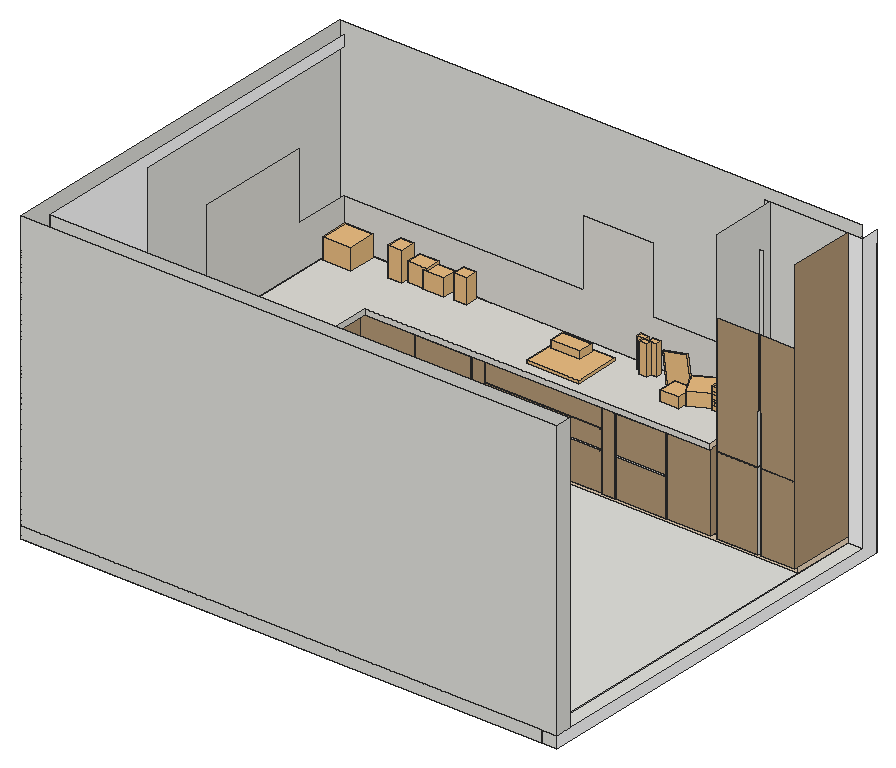
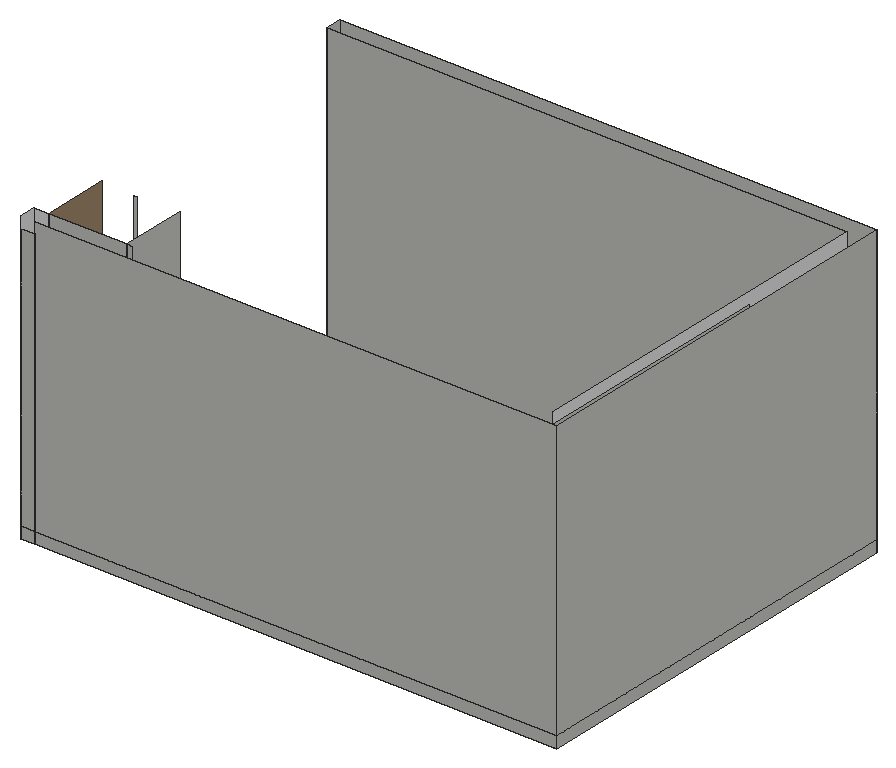
# SketchUp Ruby script. Lengths in inches.
U = 1.inch
M = Sketchup.active_model
def pt(a) = Geom::Point3d.new(a.map { |v| v * U })
def face(e, loops, mat)
  f = e.add_face(loops[0].map { |a| pt(a) })
  loops[1..].each { |l| e.add_face(l.map { |a| pt(a) }).erase! }
  f.material = f.back_material = mat if mat
  f
end
# faces: each face lists its corners as indices into pts; further lists are holes
def faces(e, pts, list, mat = nil) = list.each { |f| face(e, (f[0].is_a?(Array) ? f : [f]).map { |l| l.map { |i| pts[i] } }, mat) }
# xy, xz, yz: faces in a plane at the given z, y or x. An outline is a flat list of corners, or four numbers for a rectangle; further outlines are holes
def ring(l) = l.size == 4 ? [[l[0], l[1]], [l[2], l[1]], [l[2], l[3]], [l[0], l[3]]] : l.each_slice(2).to_a
def flat(e, list, mat, &to3) = list.each { |f| face(e, (f[0].is_a?(Array) ? f : [f]).map { |l| ring(l).map { |u, v| to3.(u, v) } }, mat) }
def xy(e, z, list, mat = nil) = flat(e, list, mat) { |x, y| [x, y, z] }
def xz(e, y, list, mat = nil) = flat(e, list, mat) { |x, z| [x, y, z] }
def yz(e, x, list, mat = nil) = flat(e, list, mat) { |y, z| [x, y, z] }
def lines(e, pts, list) = list.each { |a, b| e.add_line(pt(pts[a]), pt(pts[b])) }
# prism: a flat outline (further loops are holes) pulled along v
def prism(e, loops, v, mat = nil)
  f = face(e, loops, mat); d = Geom::Vector3d.new(v.map { |x| x * U })
  f.pushpull(f.normal.samedirection?(d) ? d.length : -d.length)
end
def box(e, o, s, mat = nil) = prism(e, [[o, [o[0] + s[0], o[1], o[2]], [o[0] + s[0], o[1] + s[1], o[2]], [o[0], o[1] + s[1], o[2]]]], [0, 0, s[2]], mat)
def at(x, y, z, deg = 0) = Geom::Transformation.translation(pt([x, y, z])) * Geom::Transformation.rotation(ORIGIN, Z_AXIS, deg.degrees)
def axes(o, x, y, z) = Geom::Transformation.new([*x, 0, *y, 0, *z, 0, *pt(o).to_a, 1])
def part(name) = M.definitions.add(name)
# library, detail: a bought-in or finely detailed component or shape, given as its bounding box
def library(name, o, s) = part(name).tap { |d| box(d.entities, o, s) }
def detail(e, o, s) = box(e.add_group.entities, o, s)
def put(e, d, t, mat = nil) = e.add_instance(d, t).tap { |i| i.material = mat if mat }
def group(e, t, mat = nil) = e.add_group.tap { |g| g.transformation = t; g.material = mat if mat }.entities
root = M.entities
M.materials.add("Generic").color = [180, 152, 118]
M.materials.add("Generic\#2").color = [244, 221, 193]
M.materials.add("Sink Modena 7170-03").color = [86, 64, 57]
M.materials.add("[Color M00]").color = [255, 255, 255]
M.materials.add("[Marble Carrara Gold Floor Tile]").color = [224, 222, 216]
M.materials.add("besi putih_Glossy3").color = [240, 240, 240]
M.materials.add("go trang").color = [128, 128, 128]
c1 = library("Group\#102",[0,0,-8.66],[20.47,15.75,8.66])
c2 = library("itchenFaucet_Handspray\#1",[0.83,4.01,0],[10.6,4,15.3])
c3 = library("Group\#11",[0,-0.59,0],[9.56,0.59,14.02])
c4 = library("Groupe\#137",[0,0,0],[2.62,1.52,5.61])
c5 = library("olive+oil",[0,0,0],[2.33,2.33,12.9])
c6 = library("bowl (2)",[-113.69,-113.69,5.71],[227.38,227.38,40.56])
c7 = library("Mixer",[2.53,2.84,0],[8.2,7.51,15.59])
c8 = library("skp23",[-4.02,-4.02,0.38],[10.21,8.04,10.27])
c9 = library("FF_Model_ID12346_3_IlluminatedPlanterCollectionLiscioCF3SU7",[0,0,0],[43.54,41.82,102.67])
c10 = library("Group\#101",[0,0,0],[12.18,12.02,6.69])
c11 = library("Group\#72",[0,0,0],[11.59,8.58,9.7])
c12 = library("Group\#138",[0,0,-0.28],[10.09,10.09,5.53])
c13 = library("kitchen",[57.57,5.21,10.61],[18.31,18.31,13.72])
c14 = library("Gas+stove+1",[-1.08,5.28,0.24],[28.08,24.69,1.54])
c15 = library("Group\#303",[-1.56,-0.52,0.97],[54.35,28.12,12.66])
c16 = library("Folded kitchen towel",[0,0,0],[1.15,10.02,12.01])
xy(root,-6,[[0,0,281.625,216],[281.625,0,289.6875,216]])
xy(root,0,[[281.625,0,289.6875,9],[9,9,281.625,9,281.625,173.25,45.375,173.25,45.375,79,9,79],[281.625,9,289.6875,207],[9,171,45.375,171,45.375,173.25,281.625,173.25,281.625,207,9,207]])
xy(root,3,[[45.375,79,46.75,105.6875],[45.375,105.6875,45.375,171,46.75,171,46.75,105.99,46.45,105.99,46.45,105.6875],[9,171,45.375,171,45.375,173.25,46.75,173.25,46.75,207,9,207],[45.375,171,46.75,173.25],[46.75,171,76.125,173.25],
  [76.43,171,79.875,171,79.875,173.25,76.125,173.25,76.125,171.3,76.43,171.3],[79.875,171,89.875,173.25],[89.875,171,106.72,171,106.72,171.3,107.02,171.3,107.02,173.25,89.875,173.25],[107.02,171,114.02,173.25],[114.33,171,161.5,171,161.5,173.25,114.02,173.25,114.02,171.3,114.33,171.3],
  [161.5,171,171.5,173.25],[171.5,171,177.3,171,177.3,171.3,177.6,171.3,177.6,173.25,171.5,173.25],[177.6,171,184.6,173.25],[184.9,171,200.1875,171,200.1875,173.25,184.6,173.25,184.6,171.3,184.9,171.3],[200.1875,171,212.05,173.25],
  [212.35,171,236.5,171,236.5,173.25,212.05,173.25,212.05,171.3,212.35,171.3],[239.5625,171,261.8125,173.25],[263.25,171,281.625,173.25],[261.8125,172.375,263.25,173.25],[46.75,173.25,79.875,207],
  [79.875,173.25,89.875,207],[89.875,173.25,161.5,207],[161.5,173.25,171.5,207],[171.5,173.25,200.1875,207],[200.1875,173.25,236.5,207],
  [236.5,173.25,239.5625,207],[239.5625,173.25,261.8125,207],[261.8125,173.25,281.625,207]])
xy(root,23.1875,[[184.9,171,212.05,171.3]])
xy(root,23.5,[[114.33,171,177.3,171.3]])
xy(root,24.1875,[[184.9,171,212.05,171.3]])
xy(root,24.5,[[114.33,171,177.3,171.3]])
xy(root,34.25,[[114.33,171,177.3,171.3]])
xy(root,34.75,[[114.33,171,177.3,171.3]])
xy(root,45.08,[[239.5625,171,261.8125,171.3],[263.25,171,281.625,171.3]])
xy(root,45.375,[[9,74.5,46.75,79],[46.75,74.5,50.25,105.6875],[[9,79,9,171,46.75,171,46.75,105.99,46.45,105.99,46.45,105.6875,46.75,105.6875,46.75,79],[18.05,81.72,36.64,103.47]],[46.45,105.6875,50.25,105.99],[46.75,105.99,50.25,169.75],
  [46.75,169.75,76.125,171],[76.125,169.75,76.43,171.3],[76.43,169.75,106.72,171],[106.72,169.75,107.02,171.3],[107.02,169.75,114.02,171],
  [114.02,169.75,114.33,171.3],[114.33,169.75,177.3,171],[177.3,169.75,177.6,171.3],[177.6,169.75,184.6,171],[184.6,169.75,184.9,171.3],
  [184.9,169.75,212.05,171],[212.05,169.75,212.35,171.3],[212.35,169.75,236.5,171],[9,171,9,207,236.5,207,236.5,171,212.35,171,212.35,171.3,212.05,171.3,212.05,171,184.9,171,184.9,171.3,184.6,171.3,184.6,171,177.6,171,177.6,171.3,177.3,171.3,177.3,171,114.33,171,114.33,171.3,114.02,171.3,114.02,171,107.02,171,107.02,171.3,106.72,171.3,106.72,171,76.43,171,76.43,171.3,76.125,171.3,76.125,171],[239.5625,171,261.8125,171.3],
  [263.25,171,281.625,171.3]])
xy(root,48.375,[[[9,74.5,50.25,74.5,50.25,169.75,236.5,169.75,236.5,207,9,207],[18.05,81.72,36.64,103.47]]],"[Marble Carrara Gold Floor Tile]")
xz(root,0,[[0,-6,281.625,0],[281.625,-6,289.6875,0],[0,0,289.6875,150]])
xz(root,9,[[9,0,289.6875,150]])
xz(root,74.5,[[9,45.375,50.25,48.375]])
xz(root,79,[[9,0,45.375,3]])
xz(root,79,[[9,3,46.75,45.375]],"Generic")
xz(root,81.72,[[18.05,45.375,36.64,48.375]])
xz(root,103.47,[[18.05,45.375,36.64,48.375]])
xz(root,105.6875,[[46.45,3,46.75,45.375]])
xz(root,105.99,[[46.45,3,46.75,45.375]])
xz(root,169.75,[[50.25,45.375,236.5,48.375]],"[Marble Carrara Gold Floor Tile]")
xz(root,171,[[9,3,46.75,45.375]])
xz(root,171,[[46.75,3,76.125,45.375],[76.43,3,106.72,45.375],[107.02,3,114.02,45.375],[114.33,3,177.3,23.5],[177.6,3,184.6,45.375],
  [184.9,3,212.05,23.1875],[212.35,3,236.5,45.375],[239.5625,3,261.8125,45.08],[263.25,3,281.625,45.08],[184.9,24.1875,212.05,45.375],
  [114.33,24.5,177.3,34.25],[114.33,34.75,177.3,45.375],[239.5625,45.375,261.8125,109.72],[263.25,45.375,281.625,109.72]],"Generic")
xz(root,171.3,[[76.125,3,76.43,45.375],[106.72,3,107.02,45.375],[114.02,3,114.33,45.375],[177.3,3,177.6,45.375],[184.6,3,184.9,45.375],
  [212.05,3,212.35,45.375],[184.9,23.1875,212.05,24.1875],[114.33,23.5,177.3,24.5],[114.33,34.25,177.3,34.75],[239.5625,45.08,261.8125,45.375],
  [263.25,45.08,281.625,45.375]])
xz(root,172.375,[[261.8125,3,263.25,150]])
xz(root,173.25,[[45.375,0,281.625,3]],"Generic\#2")
xz(root,207,[[9,0,281.625,3],[9,3,46.75,45.375],[46.75,3,79.875,45.375],[79.875,3,89.875,45.375],[89.875,3,161.5,45.375],
  [161.5,3,171.5,45.375],[171.5,3,200.1875,45.375],[200.1875,3,236.5,45.375],[236.5,3,239.5625,150],[239.5625,3,281.625,150],
  [9,45.375,46.75,48.375],[46.75,45.375,79.875,48.375],[79.875,45.375,89.875,48.375],[89.875,45.375,161.5,48.375],[161.5,45.375,171.5,48.375],
  [171.5,45.375,200.1875,48.375],[200.1875,45.375,236.5,48.375]])
xz(root,207,[[281.625,0,289.6875,150]],"[Color M00]")
xz(root,207,[[9,48.375,236.5,48.375,236.5,72,175.875,72,175.875,108,139,108,139,72,9,72]],"[Marble Carrara Gold Floor Tile]")
xz(root,216,[[0,-6,281.625,0],[281.625,-6,289.6875,0],[0,0,281.625,150],[281.625,0,289.6875,144]])
yz(root,0,[[0,-6,216,0],[0,0,216,150]])
yz(root,9,[[171,0,207,3],[171,3,207,45.375],[74.5,45.375,171,48.375],[171,45.375,207,48.375]])
yz(root,9,[[9,0,79,0,79,45.375,74.5,45.375,74.5,144,207,144,207,150,9,150]],"[Color M00]")
yz(root,9,[[74.5,48.375,207,48.375,207,72,177,72,177,108,115,108,115,72,74.5,72]],"[Marble Carrara Gold Floor Tile]")
yz(root,18.05,[[81.72,45.375,103.47,48.375]])
yz(root,36.64,[[81.72,45.375,103.47,48.375]])
yz(root,45.375,[[79,0,173.25,3]],"Generic\#2")
yz(root,46.45,[[105.6875,3,105.99,45.375]])
yz(root,46.75,[[79,3,105.6875,45.375],[105.99,3,171,45.375]],"Generic")
yz(root,50.25,[[74.5,45.375,169.75,48.375]],"[Marble Carrara Gold Floor Tile]")
yz(root,76.125,[[171,3,171.3,45.375]])
yz(root,76.43,[[171,3,171.3,45.375]])
yz(root,106.72,[[171,3,171.3,45.375]])
yz(root,107.02,[[171,3,171.3,45.375]])
yz(root,114.02,[[171,3,171.3,45.375]])
yz(root,114.33,[[171,3,171.3,23.5],[171,24.5,171.3,34.25],[171,34.75,171.3,45.375]])
yz(root,177.3,[[171,3,171.3,23.5],[171,24.5,171.3,34.25],[171,34.75,171.3,45.375]])
yz(root,177.6,[[171,3,171.3,45.375]])
yz(root,184.6,[[171,3,171.3,45.375]])
yz(root,184.9,[[171,3,171.3,23.1875],[171,24.1875,171.3,45.375]])
yz(root,212.05,[[171,3,171.3,23.1875],[171,24.1875,171.3,45.375]])
yz(root,212.35,[[171,3,171.3,45.375]])
yz(root,236.5,[[171,3,207,45.375]],"Generic")
yz(root,236.5,[[169.75,45.375,207,48.375]],"Generic\#2")
yz(root,239.5625,[[171,3,171,45.08,171.3,45.08,171.3,45.375,171,45.375,171,109.72,171.3,109.72,171.3,110.02,171,110.02,171,150,207,150,207,3]])
yz(root,261.8125,[[171,3,172.375,45.08],[171.3,45.08,172.375,45.375],[171,45.375,172.375,72]])
yz(root,263.25,[[171,3,172.375,45.08],[171.3,45.08,172.375,45.375],[171,45.375,172.375,72]])
yz(root,281.625,[[0,-6,0,0,207,0,207,144,216,144,216,-6]])
yz(root,281.625,[[171,3,207,3,207,150,171,150,171,110.02,171.3,110.02,171.3,109.72,171,109.72,171,45.375,171.3,45.375,171.3,45.08,171,45.08]],"Generic")
yz(root,281.625,[[173.25,0,207,3]],"Generic\#2")
yz(root,289.6875,[[0,0,9,150]])
yz(root,289.6875,[[0,-6,216,-6,216,150,207,150,207,0,0,0]],"[Color M00]")
p = [[106.72,171.3,45.375],[106.72,171.3,48.375],[107.02,171.3,45.375],[107.02,171.3,48.375],[114.02,171.3,45.375],[114.02,171.3,48.375],
  [114.33,171.3,45.375],[114.33,171.3,48.375],[177.3,171.3,45.375],[177.3,171.3,48.375],[177.6,171.3,45.375],[177.6,171.3,48.375],
  [184.9,171.3,45.375],[184.9,171.3,48.375],[212.05,171.3,45.375],[212.05,171.3,48.375],[212.35,171.3,45.375],[212.35,171.3,48.375],
  [46.45,105.99,45.375],[46.45,105.99,48.375],[46.75,171,45.375],[46.75,171,48.375],[184.6,171.3,45.375],[184.6,171.3,48.375],
  [46.45,105.6875,45.375],[46.45,105.6875,48.375],[46.75,169.75,45.375],[46.75,169.75,48.375]]
lines(root,p,[[0,1],[2,3],[4,5],[6,7],[8,9],[10,11],[12,13],[14,15],[16,17],[18,19],[20,21],[22,23],
  [24,25],[26,27]])
put(root,c1,axes([38.62,80.35,48.77],[0,1.15,0],[-1.3816,0,0],[0,0,1]),"Sink Modena 7170-03")
put(root,c2,axes([11.27,86.75,47.8],[0.60068,0,0],[0,1.15,0],[0,0,1]),"besi putih_Glossy3")
put(root,c3,axes([192.51,196.91,48.04],[1.2507,0.14916,0.16251],[-0.14791,1.26121,-0.01926],[-0.16365,0.00004,1.25941]))
put(root,c4,axes([11.39,82.67,48.22],[0,-2.1175,0],[2.1175,0,0],[0,0,2.1175]))
put(root,c5,axes([172.31,200.9,48.375],[1.9096,0,0],[0,1.24,0],[0,0,1.24]))
put(root,c5,axes([178.81,200.9,48.375],[1.9096,0,0],[0,1.24,0],[0,0,1.24]))
put(root,c6,axes([226.06,199.87,48.04],[0.0594,0,0],[0,0.0594,0],[0,0,0.0594]))
put(root,c7,at(51.68,194.27,48.375,90))
put(root,c8,at(54.33,202.8125,47.99))
put(root,c9,axes([74.63,199.32,48.375],[0.16,0,0],[0,0.15875,0],[0,0,0.125]),"go trang")
put(root,c10,axes([208.38,188.74,48.375],[0.98706,0.52926,0],[-0.52926,0.98706,0],[0,0,1.12]))
put(root,c11,axes([70.23,206.21,48.375],[-0.95,0,0],[0,-0.95,0],[0,0,0.95]))
put(root,c12,at(197.33,185.33,48.65))
put(root,c13,axes([-36.7,187.03,39.67],[0.82,0,0],[0,0.82,0],[0,0,0.82]))
put(root,c14,at(134.07,170.41,48.13))
put(root,c5,axes([176.18,197.46,48.75],[1.9096,0,0],[0,1.24,0],[0,0,1.24]))
put(root,c15,axes([134.85,190.28,49.87],[0.29165,0,0],[0,0.29165,0],[0,0,0.29165]))
put(root,c6,axes([226.06,199.87,49.85],[0.0594,0,0],[0,0.0594,0],[0,0,0.0594]))
put(root,c6,axes([226.06,199.87,51.66],[0.0594,0,0],[0,0.0594,0],[0,0,0.0594]))
put(root,c6,axes([226.06,199.87,53.47],[0.0594,0,0],[0,0.0594,0],[0,0,0.0594]))
put(root,c16,at(10.55,96.24,54.42),"go trang")
put(root,c6,axes([226.06,199.87,55.29],[0.0594,0,0],[0,0.0594,0],[0,0,0.0594]))
put(root,c6,axes([226.06,199.87,57.1],[0.0594,0,0],[0,0.0594,0],[0,0,0.0594]))
